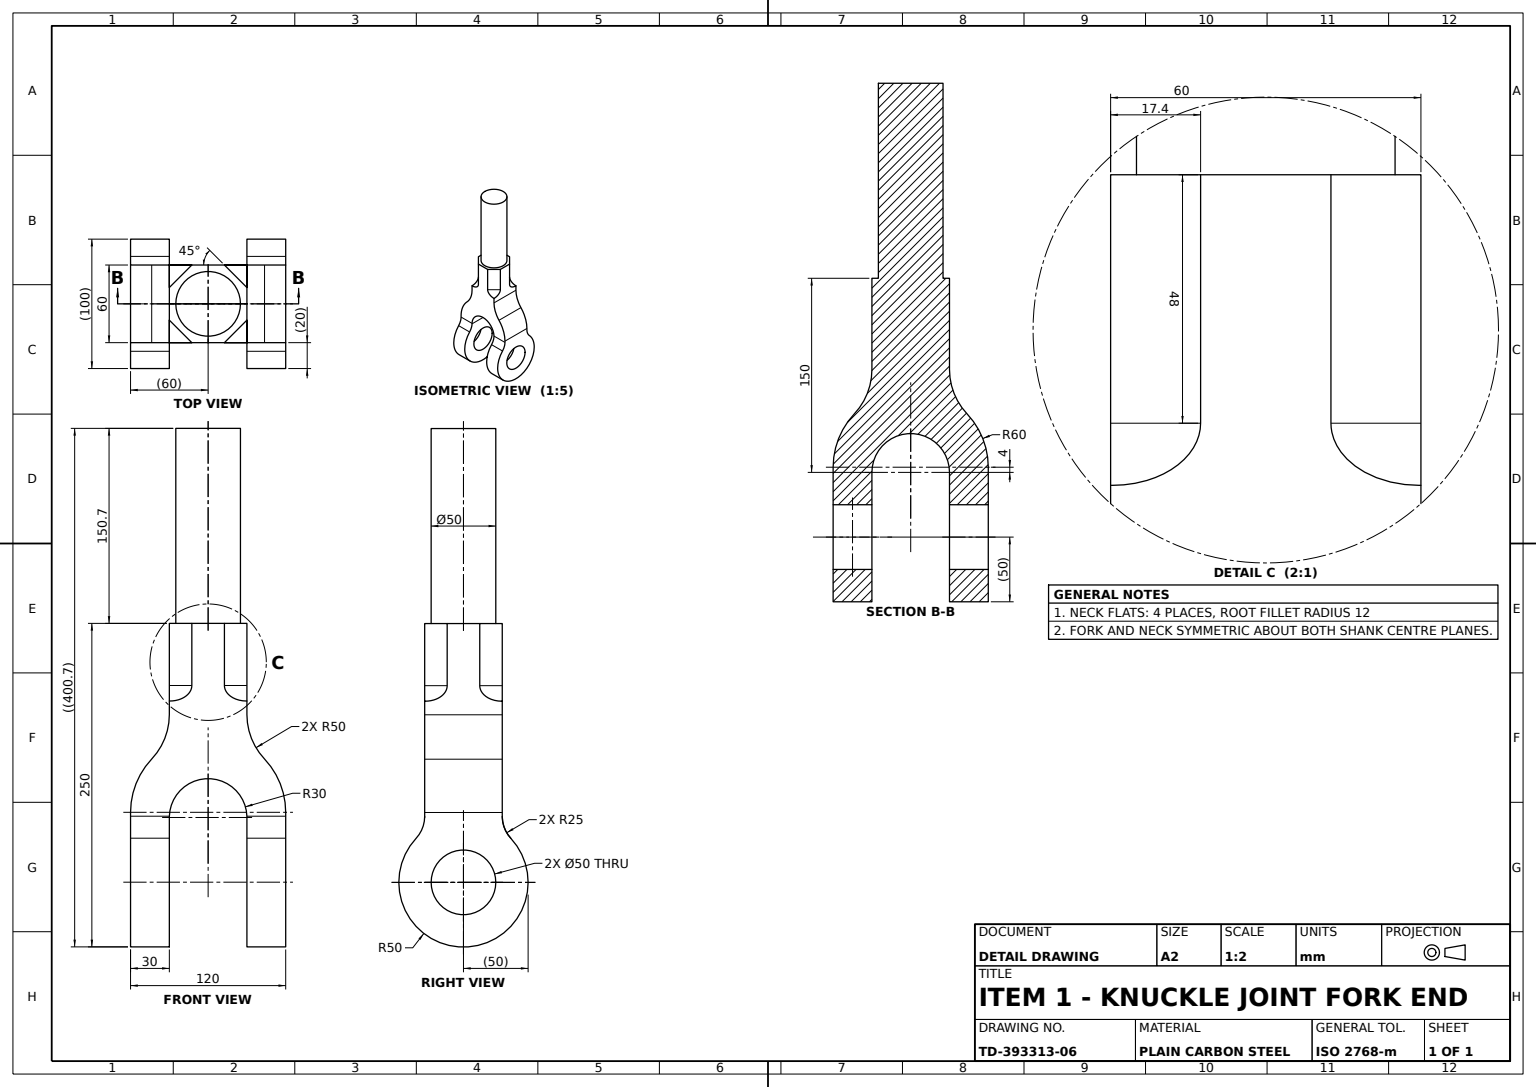
ISO-10303-21;
HEADER;
FILE_DESCRIPTION((''),'2;1');
FILE_NAME('','',(''),(''),'','','');
FILE_SCHEMA(('AUTOMOTIVE_DESIGN'));
ENDSEC;
DATA;
#1=APPLICATION_CONTEXT('');
#2=PRODUCT_CONTEXT('',#1,'mechanical');
#3=PRODUCT('','','',(#2));
#4=PRODUCT_DEFINITION_FORMATION('','',#3);
#5=PRODUCT_DEFINITION_CONTEXT('',#1,'design');
#6=PRODUCT_DEFINITION('','',#4,#5);
#7=PRODUCT_DEFINITION_SHAPE('','',#6);
#8=(LENGTH_UNIT()NAMED_UNIT(*)SI_UNIT(.MILLI.,.METRE.));
#9=(NAMED_UNIT(*)PLANE_ANGLE_UNIT()SI_UNIT($,.RADIAN.));
#10=(NAMED_UNIT(*)SI_UNIT($,.STERADIAN.)SOLID_ANGLE_UNIT());
#11=UNCERTAINTY_MEASURE_WITH_UNIT(LENGTH_MEASURE(1.E-05),#8,'distance_accuracy_value','');
#12=(GEOMETRIC_REPRESENTATION_CONTEXT(3)GLOBAL_UNCERTAINTY_ASSIGNED_CONTEXT((#11))GLOBAL_UNIT_ASSIGNED_CONTEXT((#8,#9,#10))REPRESENTATION_CONTEXT('',''));
#13=CARTESIAN_POINT('',(-90.,100.,19.980383));
#14=VERTEX_POINT('',#13);
#15=CARTESIAN_POINT('',(-90.,100.,80.019617));
#16=VERTEX_POINT('',#15);
#17=CARTESIAN_POINT('',(-90.,100.,0.));
#18=DIRECTION('',(0.,0.,1.));
#19=VECTOR('',#18,1000.);
#20=LINE('',#17,#19);
#21=EDGE_CURVE('',#14,#16,#20,.T.);
#22=ORIENTED_EDGE('',*,*,#21,.F.);
#23=CARTESIAN_POINT('',(-89.983654,100.990195,20.));
#24=VERTEX_POINT('',#23);
#25=CARTESIAN_POINT('',(-90.,100.164684,19.98691));
#26=CARTESIAN_POINT('',(-89.998644,100.329542,19.991814));
#27=CARTESIAN_POINT('',(-89.993202,100.659606,19.998359));
#28=CARTESIAN_POINT('',(-89.989107,100.825084,20.));
#29=B_SPLINE_CURVE_WITH_KNOTS('',3,(#13,#25,#26,#27,#28,#23),.UNSPECIFIED.,.F.,.F.,(4,2,4),(0.165848056,0.166335326,0.166822597),.UNSPECIFIED.);
#30=EDGE_CURVE('',#14,#24,#29,.T.);
#31=ORIENTED_EDGE('',*,*,#30,.T.);
#32=CARTESIAN_POINT('',(-30.016346,100.990195,20.));
#33=VERTEX_POINT('',#32);
#34=CARTESIAN_POINT('',(-60.,100.,20.));
#35=DIRECTION('',(0.,1.,0.));
#36=AXIS2_PLACEMENT_3D('',#34,#18,#35);
#37=CIRCLE('',#36,30.);
#38=EDGE_CURVE('',#33,#24,#37,.T.);
#39=ORIENTED_EDGE('',*,*,#38,.F.);
#40=CARTESIAN_POINT('',(-30.,100.,19.980383));
#41=VERTEX_POINT('',#40);
#42=CARTESIAN_POINT('',(-30.010903,100.82538,20.));
#43=CARTESIAN_POINT('',(-30.002731,100.495534,19.996741));
#44=CARTESIAN_POINT('',(-30.,100.165251,19.986933));
#45=B_SPLINE_CURVE_WITH_KNOTS('',3,(#32,#42,#43,#44,#40),.UNSPECIFIED.,.F.,.F.,(4,1,4),(0.085636646,0.086132211,0.086627775),.UNSPECIFIED.);
#46=EDGE_CURVE('',#33,#41,#45,.T.);
#47=ORIENTED_EDGE('',*,*,#46,.T.);
#48=CARTESIAN_POINT('',(-30.,100.,80.019617));
#49=VERTEX_POINT('',#48);
#50=CARTESIAN_POINT('',(-30.,100.,0.));
#51=LINE('',#50,#19);
#52=EDGE_CURVE('',#41,#49,#51,.T.);
#53=ORIENTED_EDGE('',*,*,#52,.T.);
#54=CARTESIAN_POINT('',(-30.016346,100.990195,80.));
#55=VERTEX_POINT('',#54);
#56=CARTESIAN_POINT('',(-30.005444,100.660091,80.));
#57=CARTESIAN_POINT('',(-30.,100.330025,80.006536));
#58=B_SPLINE_CURVE_WITH_KNOTS('',3,(#54,#56,#57,#48),.UNSPECIFIED.,.F.,.F.,(4,4),(0.,0.000990524),.UNSPECIFIED.);
#59=EDGE_CURVE('',#55,#49,#58,.T.);
#60=ORIENTED_EDGE('',*,*,#59,.F.);
#61=CARTESIAN_POINT('',(-89.983654,100.990195,80.));
#62=VERTEX_POINT('',#61);
#63=CARTESIAN_POINT('',(-60.,100.,80.));
#64=AXIS2_PLACEMENT_3D('',#63,#18,#35);
#65=CIRCLE('',#64,30.);
#66=EDGE_CURVE('',#55,#62,#65,.T.);
#67=ORIENTED_EDGE('',*,*,#66,.T.);
#68=CARTESIAN_POINT('',(-90.,100.330025,80.006536));
#69=CARTESIAN_POINT('',(-89.994556,100.660091,80.));
#70=B_SPLINE_CURVE_WITH_KNOTS('',3,(#15,#68,#69,#61),.UNSPECIFIED.,.F.,.F.,(4,4),(0.,0.000990524),.UNSPECIFIED.);
#71=EDGE_CURVE('',#16,#62,#70,.T.);
#72=ORIENTED_EDGE('',*,*,#71,.F.);
#73=EDGE_LOOP('',(#22,#31,#39,#47,#53,#60,#67,#72));
#74=FACE_OUTER_BOUND('',#73,.T.);
#75=CARTESIAN_POINT('',(-60.,100.,0.));
#76=DIRECTION('',(1.,0.,0.));
#77=AXIS2_PLACEMENT_3D('',#75,#18,#76);
#78=CYLINDRICAL_SURFACE('',#77,30.);
#79=ADVANCED_FACE('',(#74),#78,.F.);
#80=CARTESIAN_POINT('',(-120.,83.993463,86.666667));
#81=VERTEX_POINT('',#80);
#82=CARTESIAN_POINT('',(-120.,100.990195,80.));
#83=VERTEX_POINT('',#82);
#84=CARTESIAN_POINT('',(-120.,100.990195,105.));
#85=AXIS2_PLACEMENT_3D('',#84,#76,#18);
#86=CIRCLE('',#85,25.);
#87=EDGE_CURVE('',#81,#83,#86,.T.);
#88=ORIENTED_EDGE('',*,*,#87,.F.);
#89=CARTESIAN_POINT('',(-90.,83.993463,86.666667));
#90=VERTEX_POINT('',#89);
#91=CARTESIAN_POINT('',(0.,83.993463,86.666667));
#92=DIRECTION('',(-1.,0.,0.));
#93=VECTOR('',#92,1000.);
#94=LINE('',#91,#93);
#95=EDGE_CURVE('',#90,#81,#94,.T.);
#96=ORIENTED_EDGE('',*,*,#95,.F.);
#97=CARTESIAN_POINT('',(-90.,100.990195,105.));
#98=DIRECTION('',(0.,-1.,0.));
#99=AXIS2_PLACEMENT_3D('',#97,#76,#98);
#100=CIRCLE('',#99,25.);
#101=EDGE_CURVE('',#90,#16,#100,.T.);
#102=ORIENTED_EDGE('',*,*,#101,.T.);
#103=ORIENTED_EDGE('',*,*,#71,.T.);
#104=CARTESIAN_POINT('',(0.,100.990195,80.));
#105=LINE('',#104,#93);
#106=EDGE_CURVE('',#62,#83,#105,.T.);
#107=ORIENTED_EDGE('',*,*,#106,.T.);
#108=EDGE_LOOP('',(#88,#96,#102,#103,#107));
#109=FACE_OUTER_BOUND('',#108,.T.);
#110=CARTESIAN_POINT('',(0.,100.990195,105.));
#111=AXIS2_PLACEMENT_3D('',#110,#92,#18);
#112=CYLINDRICAL_SURFACE('',#111,25.);
#113=ADVANCED_FACE('',(#109),#112,.F.);
#114=CARTESIAN_POINT('',(-120.,50.,0.));
#115=VERTEX_POINT('',#114);
#116=CARTESIAN_POINT('',(-120.,50.,100.));
#117=VERTEX_POINT('',#116);
#118=CARTESIAN_POINT('',(-120.,50.,50.));
#119=AXIS2_PLACEMENT_3D('',#118,#92,#18);
#120=CIRCLE('',#119,50.);
#121=EDGE_CURVE('',#115,#117,#120,.T.);
#122=ORIENTED_EDGE('',*,*,#121,.T.);
#123=EDGE_CURVE('',#117,#81,#120,.T.);
#124=ORIENTED_EDGE('',*,*,#123,.T.);
#125=ORIENTED_EDGE('',*,*,#87,.T.);
#126=CARTESIAN_POINT('',(-120.,104.,80.));
#127=VERTEX_POINT('',#126);
#128=CARTESIAN_POINT('',(-120.,0.,80.));
#129=VECTOR('',#98,1000.);
#130=LINE('',#128,#129);
#131=EDGE_CURVE('',#127,#83,#130,.T.);
#132=ORIENTED_EDGE('',*,*,#131,.F.);
#133=CARTESIAN_POINT('',(-120.,104.,20.));
#134=VERTEX_POINT('',#133);
#135=CARTESIAN_POINT('',(-120.,104.,0.));
#136=LINE('',#135,#19);
#137=EDGE_CURVE('',#134,#127,#136,.T.);
#138=ORIENTED_EDGE('',*,*,#137,.F.);
#139=CARTESIAN_POINT('',(-120.,100.990195,20.));
#140=VERTEX_POINT('',#139);
#141=CARTESIAN_POINT('',(-120.,0.,20.));
#142=LINE('',#141,#129);
#143=EDGE_CURVE('',#134,#140,#142,.T.);
#144=ORIENTED_EDGE('',*,*,#143,.T.);
#145=CARTESIAN_POINT('',(-120.,83.993463,13.333333));
#146=VERTEX_POINT('',#145);
#147=CARTESIAN_POINT('',(-120.,100.990195,-5.));
#148=AXIS2_PLACEMENT_3D('',#147,#92,#18);
#149=CIRCLE('',#148,25.);
#150=EDGE_CURVE('',#146,#140,#149,.T.);
#151=ORIENTED_EDGE('',*,*,#150,.F.);
#152=EDGE_CURVE('',#146,#115,#120,.T.);
#153=ORIENTED_EDGE('',*,*,#152,.T.);
#154=EDGE_LOOP('',(#122,#124,#125,#132,#138,#144,#151,#153));
#155=FACE_OUTER_BOUND('',#154,.T.);
#156=CARTESIAN_POINT('',(-120.,50.,25.));
#157=VERTEX_POINT('',#156);
#158=CARTESIAN_POINT('',(-120.,50.,75.));
#159=VERTEX_POINT('',#158);
#160=CIRCLE('',#119,25.);
#161=EDGE_CURVE('',#157,#159,#160,.T.);
#162=ORIENTED_EDGE('',*,*,#161,.F.);
#163=EDGE_CURVE('',#159,#157,#160,.T.);
#164=ORIENTED_EDGE('',*,*,#163,.F.);
#165=EDGE_LOOP('',(#162,#164));
#166=FACE_BOUND('',#165,.T.);
#167=CARTESIAN_POINT('',(-120.,0.,100.));
#168=DIRECTION('',(0.,0.,-1.));
#169=AXIS2_PLACEMENT_3D('',#167,#76,#168);
#170=PLANE('',#169);
#171=ADVANCED_FACE('',(#155,#166),#170,.F.);
#172=CARTESIAN_POINT('',(-30.,250.,37.4));
#173=VERTEX_POINT('',#172);
#174=CARTESIAN_POINT('',(-47.4,250.,20.));
#175=VERTEX_POINT('',#174);
#176=CARTESIAN_POINT('',(-33.7,250.,33.7));
#177=DIRECTION('',(-0.707106781,0.,-0.707106781));
#178=VECTOR('',#177,1000.);
#179=LINE('',#176,#178);
#180=EDGE_CURVE('',#173,#175,#179,.T.);
#181=ORIENTED_EDGE('',*,*,#180,.F.);
#182=CARTESIAN_POINT('',(-30.,202.,37.4));
#183=VERTEX_POINT('',#182);
#184=CARTESIAN_POINT('',(-30.,190.,37.4));
#185=VECTOR('',#35,1000.);
#186=LINE('',#184,#185);
#187=EDGE_CURVE('',#183,#173,#186,.T.);
#188=ORIENTED_EDGE('',*,*,#187,.F.);
#189=CARTESIAN_POINT('',(-47.4,202.,20.));
#190=VERTEX_POINT('',#189);
#191=LINE('',#189,#178);
#192=EDGE_CURVE('',#183,#190,#191,.T.);
#193=ORIENTED_EDGE('',*,*,#192,.T.);
#194=CARTESIAN_POINT('',(-47.4,190.,20.));
#195=LINE('',#194,#185);
#196=EDGE_CURVE('',#190,#175,#195,.T.);
#197=ORIENTED_EDGE('',*,*,#196,.T.);
#198=EDGE_LOOP('',(#181,#188,#193,#197));
#199=FACE_OUTER_BOUND('',#198,.T.);
#200=CARTESIAN_POINT('',(-33.7,190.,33.7));
#201=DIRECTION('',(0.707106781,0.,-0.707106781));
#202=AXIS2_PLACEMENT_3D('',#200,#201,#177);
#203=PLANE('',#202);
#204=ADVANCED_FACE('',(#199),#203,.T.);
#205=CARTESIAN_POINT('',(-90.,50.,75.));
#206=VERTEX_POINT('',#205);
#207=CARTESIAN_POINT('',(0.,50.,75.));
#208=LINE('',#207,#93);
#209=EDGE_CURVE('',#206,#159,#208,.T.);
#210=ORIENTED_EDGE('',*,*,#209,.F.);
#211=CARTESIAN_POINT('',(-90.,50.,25.));
#212=VERTEX_POINT('',#211);
#213=CARTESIAN_POINT('',(-90.,50.,50.));
#214=AXIS2_PLACEMENT_3D('',#213,#92,#98);
#215=CIRCLE('',#214,25.);
#216=EDGE_CURVE('',#212,#206,#215,.T.);
#217=ORIENTED_EDGE('',*,*,#216,.F.);
#218=CARTESIAN_POINT('',(0.,50.,25.));
#219=LINE('',#218,#93);
#220=EDGE_CURVE('',#212,#157,#219,.T.);
#221=ORIENTED_EDGE('',*,*,#220,.T.);
#222=ORIENTED_EDGE('',*,*,#161,.T.);
#223=EDGE_LOOP('',(#210,#217,#221,#222));
#224=FACE_OUTER_BOUND('',#223,.T.);
#225=CARTESIAN_POINT('',(0.,50.,50.));
#226=AXIS2_PLACEMENT_3D('',#225,#92,#18);
#227=CYLINDRICAL_SURFACE('',#226,25.);
#228=ADVANCED_FACE('',(#224),#227,.F.);
#229=EDGE_CURVE('',#206,#212,#215,.T.);
#230=ORIENTED_EDGE('',*,*,#229,.F.);
#231=ORIENTED_EDGE('',*,*,#209,.T.);
#232=ORIENTED_EDGE('',*,*,#163,.T.);
#233=ORIENTED_EDGE('',*,*,#220,.F.);
#234=EDGE_LOOP('',(#230,#231,#232,#233));
#235=FACE_OUTER_BOUND('',#234,.T.);
#236=ADVANCED_FACE('',(#235),#227,.F.);
#237=CARTESIAN_POINT('',(-90.,83.993463,13.333333));
#238=VERTEX_POINT('',#237);
#239=CARTESIAN_POINT('',(-90.,100.990195,-5.));
#240=AXIS2_PLACEMENT_3D('',#239,#92,#98);
#241=CIRCLE('',#240,25.);
#242=EDGE_CURVE('',#238,#14,#241,.T.);
#243=ORIENTED_EDGE('',*,*,#242,.F.);
#244=CARTESIAN_POINT('',(0.,83.993463,13.333333));
#245=LINE('',#244,#93);
#246=EDGE_CURVE('',#238,#146,#245,.T.);
#247=ORIENTED_EDGE('',*,*,#246,.T.);
#248=ORIENTED_EDGE('',*,*,#150,.T.);
#249=CARTESIAN_POINT('',(0.,100.990195,20.));
#250=LINE('',#249,#93);
#251=EDGE_CURVE('',#24,#140,#250,.T.);
#252=ORIENTED_EDGE('',*,*,#251,.F.);
#253=ORIENTED_EDGE('',*,*,#30,.F.);
#254=EDGE_LOOP('',(#243,#247,#248,#252,#253));
#255=FACE_OUTER_BOUND('',#254,.T.);
#256=CARTESIAN_POINT('',(0.,100.990195,-5.));
#257=AXIS2_PLACEMENT_3D('',#256,#92,#18);
#258=CYLINDRICAL_SURFACE('',#257,25.);
#259=ADVANCED_FACE('',(#255),#258,.F.);
#260=CARTESIAN_POINT('',(-47.4,202.,80.));
#261=VERTEX_POINT('',#260);
#262=CARTESIAN_POINT('',(-30.,202.,62.6));
#263=VERTEX_POINT('',#262);
#264=VECTOR('',#201,1000.);
#265=LINE('',#262,#264);
#266=EDGE_CURVE('',#261,#263,#265,.T.);
#267=ORIENTED_EDGE('',*,*,#266,.F.);
#268=CARTESIAN_POINT('',(-30.429437,190.,80.));
#269=VERTEX_POINT('',#268);
#270=CARTESIAN_POINT('',(-40.370563,190.,80.));
#271=CARTESIAN_POINT('',(-47.4,194.970563,80.));
#272=(BOUNDED_CURVE()B_SPLINE_CURVE(3,(#268,#270,#271,#260),.UNSPECIFIED.,.F.,.F.)B_SPLINE_CURVE_WITH_KNOTS((4,4),(4.71238898,6.283185307),.UNSPECIFIED.)CURVE()GEOMETRIC_REPRESENTATION_ITEM()RATIONAL_B_SPLINE_CURVE((1.,0.804737854,0.804737854,1.))REPRESENTATION_ITEM(''));
#273=EDGE_CURVE('',#269,#261,#272,.T.);
#274=ORIENTED_EDGE('',*,*,#273,.F.);
#275=CARTESIAN_POINT('',(-30.,190.,79.570563));
#276=VERTEX_POINT('',#275);
#277=CARTESIAN_POINT('',(-38.914719,190.,88.485281));
#278=DIRECTION('',(-0.707106781,0.,0.707106781));
#279=VECTOR('',#278,1000.);
#280=LINE('',#277,#279);
#281=EDGE_CURVE('',#276,#269,#280,.T.);
#282=ORIENTED_EDGE('',*,*,#281,.F.);
#283=CARTESIAN_POINT('',(-30.,194.970563,62.6));
#284=CARTESIAN_POINT('',(-30.,190.,69.629437));
#285=(BOUNDED_CURVE()B_SPLINE_CURVE(3,(#262,#283,#284,#275),.UNSPECIFIED.,.F.,.F.)B_SPLINE_CURVE_WITH_KNOTS((4,4),(3.141592654,4.71238898),.UNSPECIFIED.)CURVE()GEOMETRIC_REPRESENTATION_ITEM()RATIONAL_B_SPLINE_CURVE((1.,0.804737854,0.804737854,1.))REPRESENTATION_ITEM(''));
#286=EDGE_CURVE('',#263,#276,#285,.T.);
#287=ORIENTED_EDGE('',*,*,#286,.F.);
#288=EDGE_LOOP('',(#267,#274,#282,#287));
#289=FACE_OUTER_BOUND('',#288,.T.);
#290=CARTESIAN_POINT('',(24.785281,202.,24.785281));
#291=DIRECTION('',(0.707106781,0.,0.707106781));
#292=AXIS2_PLACEMENT_3D('',#290,#278,#291);
#293=CYLINDRICAL_SURFACE('',#292,12.);
#294=ADVANCED_FACE('',(#289),#293,.F.);
#295=CARTESIAN_POINT('',(-35.,400.7,50.));
#296=VERTEX_POINT('',#295);
#297=CARTESIAN_POINT('',(-85.,400.7,50.));
#298=VERTEX_POINT('',#297);
#299=CARTESIAN_POINT('',(-60.,400.7,50.));
#300=AXIS2_PLACEMENT_3D('',#299,#35,#92);
#301=CIRCLE('',#300,25.);
#302=EDGE_CURVE('',#296,#298,#301,.T.);
#303=ORIENTED_EDGE('',*,*,#302,.F.);
#304=CARTESIAN_POINT('',(-35.,250.,50.));
#305=VERTEX_POINT('',#304);
#306=LINE('',#295,#129);
#307=EDGE_CURVE('',#296,#305,#306,.T.);
#308=ORIENTED_EDGE('',*,*,#307,.T.);
#309=CARTESIAN_POINT('',(-85.,250.,50.));
#310=VERTEX_POINT('',#309);
#311=CARTESIAN_POINT('',(-60.,250.,50.));
#312=AXIS2_PLACEMENT_3D('',#311,#35,#92);
#313=CIRCLE('',#312,25.);
#314=EDGE_CURVE('',#305,#310,#313,.T.);
#315=ORIENTED_EDGE('',*,*,#314,.T.);
#316=LINE('',#297,#129);
#317=EDGE_CURVE('',#298,#310,#316,.T.);
#318=ORIENTED_EDGE('',*,*,#317,.F.);
#319=EDGE_LOOP('',(#303,#308,#315,#318));
#320=FACE_OUTER_BOUND('',#319,.T.);
#321=AXIS2_PLACEMENT_3D('',#299,#98,#76);
#322=CYLINDRICAL_SURFACE('',#321,25.);
#323=ADVANCED_FACE('',(#320),#322,.T.);
#324=CARTESIAN_POINT('',(-90.,190.,79.570563));
#325=VERTEX_POINT('',#324);
#326=CARTESIAN_POINT('',(-90.,190.,80.));
#327=VERTEX_POINT('',#326);
#328=CARTESIAN_POINT('',(-90.,190.,0.));
#329=LINE('',#328,#19);
#330=EDGE_CURVE('',#325,#327,#329,.T.);
#331=ORIENTED_EDGE('',*,*,#330,.T.);
#332=CARTESIAN_POINT('',(-89.570563,190.,80.));
#333=VERTEX_POINT('',#332);
#334=CARTESIAN_POINT('',(0.,190.,80.));
#335=VECTOR('',#76,1000.);
#336=LINE('',#334,#335);
#337=EDGE_CURVE('',#327,#333,#336,.T.);
#338=ORIENTED_EDGE('',*,*,#337,.T.);
#339=CARTESIAN_POINT('',(-98.485281,190.,71.085281));
#340=LINE('',#339,#178);
#341=EDGE_CURVE('',#333,#325,#340,.T.);
#342=ORIENTED_EDGE('',*,*,#341,.T.);
#343=EDGE_LOOP('',(#331,#338,#342));
#344=FACE_OUTER_BOUND('',#343,.T.);
#345=CARTESIAN_POINT('',(0.,190.,0.));
#346=AXIS2_PLACEMENT_3D('',#345,#35,#92);
#347=PLANE('',#346);
#348=ADVANCED_FACE('',(#344),#347,.T.);
#349=CARTESIAN_POINT('',(-90.,190.,20.429437));
#350=VERTEX_POINT('',#349);
#351=CARTESIAN_POINT('',(-89.570563,190.,20.));
#352=VERTEX_POINT('',#351);
#353=CARTESIAN_POINT('',(-81.085281,190.,11.514719));
#354=LINE('',#353,#264);
#355=EDGE_CURVE('',#350,#352,#354,.T.);
#356=ORIENTED_EDGE('',*,*,#355,.T.);
#357=CARTESIAN_POINT('',(-90.,190.,20.));
#358=VERTEX_POINT('',#357);
#359=CARTESIAN_POINT('',(0.,190.,20.));
#360=LINE('',#359,#93);
#361=EDGE_CURVE('',#352,#358,#360,.T.);
#362=ORIENTED_EDGE('',*,*,#361,.T.);
#363=EDGE_CURVE('',#358,#350,#329,.T.);
#364=ORIENTED_EDGE('',*,*,#363,.T.);
#365=EDGE_LOOP('',(#356,#362,#364));
#366=FACE_OUTER_BOUND('',#365,.T.);
#367=ADVANCED_FACE('',(#366),#347,.T.);
#368=ORIENTED_EDGE('',*,*,#281,.T.);
#369=CARTESIAN_POINT('',(-30.,190.,80.));
#370=VERTEX_POINT('',#369);
#371=EDGE_CURVE('',#269,#370,#336,.T.);
#372=ORIENTED_EDGE('',*,*,#371,.T.);
#373=CARTESIAN_POINT('',(-30.,190.,0.));
#374=VECTOR('',#168,1000.);
#375=LINE('',#373,#374);
#376=EDGE_CURVE('',#370,#276,#375,.T.);
#377=ORIENTED_EDGE('',*,*,#376,.T.);
#378=EDGE_LOOP('',(#368,#372,#377));
#379=FACE_OUTER_BOUND('',#378,.T.);
#380=ADVANCED_FACE('',(#379),#347,.T.);
#381=ORIENTED_EDGE('',*,*,#46,.F.);
#382=VERTEX_POINT('',#249);
#383=EDGE_CURVE('',#382,#33,#250,.T.);
#384=ORIENTED_EDGE('',*,*,#383,.F.);
#385=VERTEX_POINT('',#244);
#386=CIRCLE('',#257,25.);
#387=EDGE_CURVE('',#385,#382,#386,.T.);
#388=ORIENTED_EDGE('',*,*,#387,.F.);
#389=CARTESIAN_POINT('',(-30.,83.993463,13.333333));
#390=VERTEX_POINT('',#389);
#391=EDGE_CURVE('',#385,#390,#245,.T.);
#392=ORIENTED_EDGE('',*,*,#391,.T.);
#393=CARTESIAN_POINT('',(-30.,100.990195,-5.));
#394=AXIS2_PLACEMENT_3D('',#393,#92,#98);
#395=CIRCLE('',#394,25.);
#396=EDGE_CURVE('',#390,#41,#395,.T.);
#397=ORIENTED_EDGE('',*,*,#396,.T.);
#398=EDGE_LOOP('',(#381,#384,#388,#392,#397));
#399=FACE_OUTER_BOUND('',#398,.T.);
#400=ADVANCED_FACE('',(#399),#258,.F.);
#401=CARTESIAN_POINT('',(-30.,50.,25.));
#402=VERTEX_POINT('',#401);
#403=CARTESIAN_POINT('',(-30.,50.,75.));
#404=VERTEX_POINT('',#403);
#405=CARTESIAN_POINT('',(-30.,50.,50.));
#406=AXIS2_PLACEMENT_3D('',#405,#92,#98);
#407=CIRCLE('',#406,25.);
#408=EDGE_CURVE('',#402,#404,#407,.T.);
#409=ORIENTED_EDGE('',*,*,#408,.F.);
#410=EDGE_CURVE('',#404,#402,#407,.T.);
#411=ORIENTED_EDGE('',*,*,#410,.F.);
#412=EDGE_LOOP('',(#409,#411));
#413=FACE_BOUND('',#412,.T.);
#414=CARTESIAN_POINT('',(-30.,50.,0.));
#415=VERTEX_POINT('',#414);
#416=CIRCLE('',#406,50.);
#417=EDGE_CURVE('',#390,#415,#416,.T.);
#418=ORIENTED_EDGE('',*,*,#417,.T.);
#419=CARTESIAN_POINT('',(-30.,50.,100.));
#420=VERTEX_POINT('',#419);
#421=EDGE_CURVE('',#415,#420,#416,.T.);
#422=ORIENTED_EDGE('',*,*,#421,.T.);
#423=CARTESIAN_POINT('',(-30.,83.993463,86.666667));
#424=VERTEX_POINT('',#423);
#425=EDGE_CURVE('',#420,#424,#416,.T.);
#426=ORIENTED_EDGE('',*,*,#425,.T.);
#427=CARTESIAN_POINT('',(-30.,100.990195,105.));
#428=AXIS2_PLACEMENT_3D('',#427,#76,#98);
#429=CIRCLE('',#428,25.);
#430=EDGE_CURVE('',#424,#49,#429,.T.);
#431=ORIENTED_EDGE('',*,*,#430,.T.);
#432=ORIENTED_EDGE('',*,*,#52,.F.);
#433=ORIENTED_EDGE('',*,*,#396,.F.);
#434=EDGE_LOOP('',(#418,#422,#426,#431,#432,#433));
#435=FACE_OUTER_BOUND('',#434,.T.);
#436=CARTESIAN_POINT('',(-30.,0.,0.));
#437=AXIS2_PLACEMENT_3D('',#436,#92,#98);
#438=PLANE('',#437);
#439=ADVANCED_FACE('',(#413,#435),#438,.T.);
#440=CARTESIAN_POINT('',(-90.,50.,0.));
#441=VERTEX_POINT('',#440);
#442=CARTESIAN_POINT('',(0.,50.,0.));
#443=LINE('',#442,#93);
#444=EDGE_CURVE('',#441,#115,#443,.T.);
#445=ORIENTED_EDGE('',*,*,#444,.F.);
#446=CARTESIAN_POINT('',(-90.,50.,100.));
#447=VERTEX_POINT('',#446);
#448=CIRCLE('',#214,50.);
#449=EDGE_CURVE('',#441,#447,#448,.T.);
#450=ORIENTED_EDGE('',*,*,#449,.T.);
#451=CARTESIAN_POINT('',(0.,50.,100.));
#452=LINE('',#451,#93);
#453=EDGE_CURVE('',#447,#117,#452,.T.);
#454=ORIENTED_EDGE('',*,*,#453,.T.);
#455=ORIENTED_EDGE('',*,*,#121,.F.);
#456=EDGE_LOOP('',(#445,#450,#454,#455));
#457=FACE_OUTER_BOUND('',#456,.T.);
#458=CYLINDRICAL_SURFACE('',#226,50.);
#459=ADVANCED_FACE('',(#457),#458,.T.);
#460=ORIENTED_EDGE('',*,*,#408,.T.);
#461=VERTEX_POINT('',#207);
#462=EDGE_CURVE('',#461,#404,#208,.T.);
#463=ORIENTED_EDGE('',*,*,#462,.F.);
#464=VERTEX_POINT('',#218);
#465=CIRCLE('',#226,25.);
#466=EDGE_CURVE('',#464,#461,#465,.T.);
#467=ORIENTED_EDGE('',*,*,#466,.F.);
#468=EDGE_CURVE('',#464,#402,#219,.T.);
#469=ORIENTED_EDGE('',*,*,#468,.T.);
#470=EDGE_LOOP('',(#460,#463,#467,#469));
#471=FACE_OUTER_BOUND('',#470,.T.);
#472=ADVANCED_FACE('',(#471),#227,.F.);
#473=VERTEX_POINT('',#442);
#474=EDGE_CURVE('',#473,#415,#443,.T.);
#475=ORIENTED_EDGE('',*,*,#474,.F.);
#476=VERTEX_POINT('',#451);
#477=CIRCLE('',#226,50.);
#478=EDGE_CURVE('',#473,#476,#477,.T.);
#479=ORIENTED_EDGE('',*,*,#478,.T.);
#480=EDGE_CURVE('',#476,#420,#452,.T.);
#481=ORIENTED_EDGE('',*,*,#480,.T.);
#482=ORIENTED_EDGE('',*,*,#421,.F.);
#483=EDGE_LOOP('',(#475,#479,#481,#482));
#484=FACE_OUTER_BOUND('',#483,.T.);
#485=ADVANCED_FACE('',(#484),#458,.T.);
#486=VERTEX_POINT('',#91);
#487=VERTEX_POINT('',#104);
#488=AXIS2_PLACEMENT_3D('',#110,#76,#18);
#489=CIRCLE('',#488,25.);
#490=EDGE_CURVE('',#486,#487,#489,.T.);
#491=ORIENTED_EDGE('',*,*,#490,.T.);
#492=EDGE_CURVE('',#487,#55,#105,.T.);
#493=ORIENTED_EDGE('',*,*,#492,.T.);
#494=ORIENTED_EDGE('',*,*,#59,.T.);
#495=ORIENTED_EDGE('',*,*,#430,.F.);
#496=EDGE_CURVE('',#486,#424,#94,.T.);
#497=ORIENTED_EDGE('',*,*,#496,.F.);
#498=EDGE_LOOP('',(#491,#493,#494,#495,#497));
#499=FACE_OUTER_BOUND('',#498,.T.);
#500=ADVANCED_FACE('',(#499),#112,.F.);
#501=CARTESIAN_POINT('',(-30.,179.498344,80.));
#502=VERTEX_POINT('',#501);
#503=CARTESIAN_POINT('',(-16.363636,145.180915,80.));
#504=VERTEX_POINT('',#503);
#505=CARTESIAN_POINT('',(20.,179.498344,80.));
#506=AXIS2_PLACEMENT_3D('',#505,#18,#35);
#507=CIRCLE('',#506,50.);
#508=EDGE_CURVE('',#502,#504,#507,.T.);
#509=ORIENTED_EDGE('',*,*,#508,.F.);
#510=CARTESIAN_POINT('',(-30.,0.,80.));
#511=LINE('',#510,#129);
#512=EDGE_CURVE('',#370,#502,#511,.T.);
#513=ORIENTED_EDGE('',*,*,#512,.F.);
#514=ORIENTED_EDGE('',*,*,#371,.F.);
#515=ORIENTED_EDGE('',*,*,#273,.T.);
#516=CARTESIAN_POINT('',(-47.4,250.,80.));
#517=VERTEX_POINT('',#516);
#518=CARTESIAN_POINT('',(-47.4,190.,80.));
#519=LINE('',#518,#185);
#520=EDGE_CURVE('',#261,#517,#519,.T.);
#521=ORIENTED_EDGE('',*,*,#520,.T.);
#522=CARTESIAN_POINT('',(-72.6,250.,80.));
#523=VERTEX_POINT('',#522);
#524=CARTESIAN_POINT('',(0.,250.,80.));
#525=LINE('',#524,#93);
#526=EDGE_CURVE('',#517,#523,#525,.T.);
#527=ORIENTED_EDGE('',*,*,#526,.T.);
#528=CARTESIAN_POINT('',(-72.6,202.,80.));
#529=VERTEX_POINT('',#528);
#530=CARTESIAN_POINT('',(-72.6,190.,80.));
#531=LINE('',#530,#185);
#532=EDGE_CURVE('',#529,#523,#531,.T.);
#533=ORIENTED_EDGE('',*,*,#532,.F.);
#534=CARTESIAN_POINT('',(-72.6,194.970563,80.));
#535=CARTESIAN_POINT('',(-79.629437,190.,80.));
#536=(BOUNDED_CURVE()B_SPLINE_CURVE(3,(#528,#534,#535,#332),.UNSPECIFIED.,.F.,.T.)B_SPLINE_CURVE_WITH_KNOTS((4,4),(3.141592654,4.71238898),.UNSPECIFIED.)CURVE()GEOMETRIC_REPRESENTATION_ITEM()RATIONAL_B_SPLINE_CURVE((1.,0.804737854,0.804737854,1.))REPRESENTATION_ITEM(''));
#537=EDGE_CURVE('',#529,#333,#536,.T.);
#538=ORIENTED_EDGE('',*,*,#537,.T.);
#539=ORIENTED_EDGE('',*,*,#337,.F.);
#540=CARTESIAN_POINT('',(-90.,179.498344,80.));
#541=VERTEX_POINT('',#540);
#542=CARTESIAN_POINT('',(-90.,0.,80.));
#543=LINE('',#542,#129);
#544=EDGE_CURVE('',#327,#541,#543,.T.);
#545=ORIENTED_EDGE('',*,*,#544,.T.);
#546=CARTESIAN_POINT('',(-103.636364,145.180915,80.));
#547=VERTEX_POINT('',#546);
#548=CARTESIAN_POINT('',(-140.,179.498344,80.));
#549=AXIS2_PLACEMENT_3D('',#548,#168,#35);
#550=CIRCLE('',#549,50.);
#551=EDGE_CURVE('',#541,#547,#550,.T.);
#552=ORIENTED_EDGE('',*,*,#551,.T.);
#553=CARTESIAN_POINT('',(-60.,104.,80.));
#554=AXIS2_PLACEMENT_3D('',#553,#18,#35);
#555=CIRCLE('',#554,60.);
#556=EDGE_CURVE('',#547,#127,#555,.T.);
#557=ORIENTED_EDGE('',*,*,#556,.T.);
#558=ORIENTED_EDGE('',*,*,#131,.T.);
#559=ORIENTED_EDGE('',*,*,#106,.F.);
#560=ORIENTED_EDGE('',*,*,#66,.F.);
#561=ORIENTED_EDGE('',*,*,#492,.F.);
#562=CARTESIAN_POINT('',(0.,104.,80.));
#563=VERTEX_POINT('',#562);
#564=CARTESIAN_POINT('',(0.,0.,80.));
#565=LINE('',#564,#129);
#566=EDGE_CURVE('',#563,#487,#565,.T.);
#567=ORIENTED_EDGE('',*,*,#566,.F.);
#568=EDGE_CURVE('',#563,#504,#555,.T.);
#569=ORIENTED_EDGE('',*,*,#568,.T.);
#570=EDGE_LOOP('',(#509,#513,#514,#515,#521,#527,#533,#538,#539,#545,#552,#557,#558,#559,#560,#561,#567,#569));
#571=FACE_OUTER_BOUND('',#570,.T.);
#572=AXIS2_PLACEMENT_3D('',#564,#168,#35);
#573=PLANE('',#572);
#574=ADVANCED_FACE('',(#571),#573,.F.);
#575=CARTESIAN_POINT('',(-16.363636,145.180915,20.));
#576=VERTEX_POINT('',#575);
#577=CARTESIAN_POINT('',(-16.363636,145.180915,0.));
#578=LINE('',#577,#19);
#579=EDGE_CURVE('',#576,#504,#578,.T.);
#580=ORIENTED_EDGE('',*,*,#579,.T.);
#581=ORIENTED_EDGE('',*,*,#568,.F.);
#582=CARTESIAN_POINT('',(0.,104.,20.));
#583=VERTEX_POINT('',#582);
#584=CARTESIAN_POINT('',(0.,104.,0.));
#585=LINE('',#584,#19);
#586=EDGE_CURVE('',#583,#563,#585,.T.);
#587=ORIENTED_EDGE('',*,*,#586,.F.);
#588=CARTESIAN_POINT('',(-60.,104.,20.));
#589=AXIS2_PLACEMENT_3D('',#588,#18,#35);
#590=CIRCLE('',#589,60.);
#591=EDGE_CURVE('',#583,#576,#590,.T.);
#592=ORIENTED_EDGE('',*,*,#591,.T.);
#593=EDGE_LOOP('',(#580,#581,#587,#592));
#594=FACE_OUTER_BOUND('',#593,.T.);
#595=CARTESIAN_POINT('',(-60.,104.,0.));
#596=AXIS2_PLACEMENT_3D('',#595,#18,#76);
#597=CYLINDRICAL_SURFACE('',#596,60.);
#598=ADVANCED_FACE('',(#594),#597,.T.);
#599=CARTESIAN_POINT('',(-72.6,202.,20.));
#600=VERTEX_POINT('',#599);
#601=CARTESIAN_POINT('',(-79.629437,190.,20.));
#602=CARTESIAN_POINT('',(-72.6,194.970563,20.));
#603=(BOUNDED_CURVE()B_SPLINE_CURVE(3,(#351,#601,#602,#599),.UNSPECIFIED.,.F.,.F.)B_SPLINE_CURVE_WITH_KNOTS((4,4),(4.71238898,6.283185307),.UNSPECIFIED.)CURVE()GEOMETRIC_REPRESENTATION_ITEM()RATIONAL_B_SPLINE_CURVE((1.,0.804737854,0.804737854,1.))REPRESENTATION_ITEM(''));
#604=EDGE_CURVE('',#352,#600,#603,.T.);
#605=ORIENTED_EDGE('',*,*,#604,.F.);
#606=ORIENTED_EDGE('',*,*,#355,.F.);
#607=CARTESIAN_POINT('',(-90.,202.,37.4));
#608=VERTEX_POINT('',#607);
#609=CARTESIAN_POINT('',(-90.,194.970563,37.4));
#610=CARTESIAN_POINT('',(-90.,190.,30.370563));
#611=(BOUNDED_CURVE()B_SPLINE_CURVE(3,(#607,#609,#610,#349),.UNSPECIFIED.,.F.,.T.)B_SPLINE_CURVE_WITH_KNOTS((4,4),(3.141592654,4.71238898),.UNSPECIFIED.)CURVE()GEOMETRIC_REPRESENTATION_ITEM()RATIONAL_B_SPLINE_CURVE((1.,0.804737854,0.804737854,1.))REPRESENTATION_ITEM(''));
#612=EDGE_CURVE('',#608,#350,#611,.T.);
#613=ORIENTED_EDGE('',*,*,#612,.F.);
#614=LINE('',#607,#279);
#615=EDGE_CURVE('',#600,#608,#614,.T.);
#616=ORIENTED_EDGE('',*,*,#615,.F.);
#617=EDGE_LOOP('',(#605,#606,#613,#616));
#618=FACE_OUTER_BOUND('',#617,.T.);
#619=CARTESIAN_POINT('',(-34.785281,202.,-34.785281));
#620=AXIS2_PLACEMENT_3D('',#619,#201,#177);
#621=CYLINDRICAL_SURFACE('',#620,12.);
#622=ADVANCED_FACE('',(#618),#621,.F.);
#623=ORIENTED_EDGE('',*,*,#462,.T.);
#624=ORIENTED_EDGE('',*,*,#410,.T.);
#625=ORIENTED_EDGE('',*,*,#468,.F.);
#626=EDGE_CURVE('',#461,#464,#465,.T.);
#627=ORIENTED_EDGE('',*,*,#626,.F.);
#628=EDGE_LOOP('',(#623,#624,#625,#627));
#629=FACE_OUTER_BOUND('',#628,.T.);
#630=ADVANCED_FACE('',(#629),#227,.F.);
#631=CARTESIAN_POINT('',(-30.,190.,20.));
#632=VERTEX_POINT('',#631);
#633=CARTESIAN_POINT('',(-30.429437,190.,20.));
#634=VERTEX_POINT('',#633);
#635=EDGE_CURVE('',#632,#634,#360,.T.);
#636=ORIENTED_EDGE('',*,*,#635,.T.);
#637=CARTESIAN_POINT('',(-30.,190.,20.429437));
#638=VERTEX_POINT('',#637);
#639=CARTESIAN_POINT('',(-21.514719,190.,28.914719));
#640=VECTOR('',#291,1000.);
#641=LINE('',#639,#640);
#642=EDGE_CURVE('',#634,#638,#641,.T.);
#643=ORIENTED_EDGE('',*,*,#642,.T.);
#644=EDGE_CURVE('',#638,#632,#375,.T.);
#645=ORIENTED_EDGE('',*,*,#644,.T.);
#646=EDGE_LOOP('',(#636,#643,#645));
#647=FACE_OUTER_BOUND('',#646,.T.);
#648=ADVANCED_FACE('',(#647),#347,.T.);
#649=CARTESIAN_POINT('',(-30.,190.,30.370563));
#650=CARTESIAN_POINT('',(-30.,194.970563,37.4));
#651=(BOUNDED_CURVE()B_SPLINE_CURVE(3,(#637,#649,#650,#182),.UNSPECIFIED.,.F.,.F.)B_SPLINE_CURVE_WITH_KNOTS((4,4),(4.71238898,6.283185307),.UNSPECIFIED.)CURVE()GEOMETRIC_REPRESENTATION_ITEM()RATIONAL_B_SPLINE_CURVE((1.,0.804737854,0.804737854,1.))REPRESENTATION_ITEM(''));
#652=EDGE_CURVE('',#638,#183,#651,.T.);
#653=ORIENTED_EDGE('',*,*,#652,.F.);
#654=ORIENTED_EDGE('',*,*,#642,.F.);
#655=CARTESIAN_POINT('',(-47.4,194.970563,20.));
#656=CARTESIAN_POINT('',(-40.370563,190.,20.));
#657=(BOUNDED_CURVE()B_SPLINE_CURVE(3,(#189,#655,#656,#633),.UNSPECIFIED.,.F.,.F.)B_SPLINE_CURVE_WITH_KNOTS((4,4),(3.141592654,4.71238898),.UNSPECIFIED.)CURVE()GEOMETRIC_REPRESENTATION_ITEM()RATIONAL_B_SPLINE_CURVE((1.,0.804737854,0.804737854,1.))REPRESENTATION_ITEM(''));
#658=EDGE_CURVE('',#190,#634,#657,.T.);
#659=ORIENTED_EDGE('',*,*,#658,.F.);
#660=ORIENTED_EDGE('',*,*,#192,.F.);
#661=EDGE_LOOP('',(#653,#654,#659,#660));
#662=FACE_OUTER_BOUND('',#661,.T.);
#663=CARTESIAN_POINT('',(-25.214719,202.,25.214719));
#664=AXIS2_PLACEMENT_3D('',#663,#291,#201);
#665=CYLINDRICAL_SURFACE('',#664,12.);
#666=ADVANCED_FACE('',(#662),#665,.F.);
#667=EDGE_CURVE('',#476,#486,#477,.T.);
#668=ORIENTED_EDGE('',*,*,#667,.T.);
#669=ORIENTED_EDGE('',*,*,#496,.T.);
#670=ORIENTED_EDGE('',*,*,#425,.F.);
#671=ORIENTED_EDGE('',*,*,#480,.F.);
#672=EDGE_LOOP('',(#668,#669,#670,#671));
#673=FACE_OUTER_BOUND('',#672,.T.);
#674=ADVANCED_FACE('',(#673),#458,.T.);
#675=ORIENTED_EDGE('',*,*,#579,.F.);
#676=CARTESIAN_POINT('',(-30.,179.498344,20.));
#677=VERTEX_POINT('',#676);
#678=CARTESIAN_POINT('',(20.,179.498344,20.));
#679=AXIS2_PLACEMENT_3D('',#678,#18,#35);
#680=CIRCLE('',#679,50.);
#681=EDGE_CURVE('',#677,#576,#680,.T.);
#682=ORIENTED_EDGE('',*,*,#681,.F.);
#683=CARTESIAN_POINT('',(-30.,179.498344,0.));
#684=LINE('',#683,#19);
#685=EDGE_CURVE('',#677,#502,#684,.T.);
#686=ORIENTED_EDGE('',*,*,#685,.T.);
#687=ORIENTED_EDGE('',*,*,#508,.T.);
#688=EDGE_LOOP('',(#675,#682,#686,#687));
#689=FACE_OUTER_BOUND('',#688,.T.);
#690=CARTESIAN_POINT('',(20.,179.498344,0.));
#691=AXIS2_PLACEMENT_3D('',#690,#18,#76);
#692=CYLINDRICAL_SURFACE('',#691,50.);
#693=ADVANCED_FACE('',(#689),#692,.F.);
#694=CARTESIAN_POINT('',(-103.636364,145.180915,20.));
#695=VERTEX_POINT('',#694);
#696=EDGE_CURVE('',#695,#134,#590,.T.);
#697=ORIENTED_EDGE('',*,*,#696,.T.);
#698=ORIENTED_EDGE('',*,*,#137,.T.);
#699=ORIENTED_EDGE('',*,*,#556,.F.);
#700=CARTESIAN_POINT('',(-103.636364,145.180915,0.));
#701=LINE('',#700,#19);
#702=EDGE_CURVE('',#695,#547,#701,.T.);
#703=ORIENTED_EDGE('',*,*,#702,.F.);
#704=EDGE_LOOP('',(#697,#698,#699,#703));
#705=FACE_OUTER_BOUND('',#704,.T.);
#706=ADVANCED_FACE('',(#705),#597,.T.);
#707=ORIENTED_EDGE('',*,*,#307,.F.);
#708=EDGE_CURVE('',#298,#296,#301,.T.);
#709=ORIENTED_EDGE('',*,*,#708,.F.);
#710=ORIENTED_EDGE('',*,*,#317,.T.);
#711=EDGE_CURVE('',#310,#305,#313,.T.);
#712=ORIENTED_EDGE('',*,*,#711,.T.);
#713=EDGE_LOOP('',(#707,#709,#710,#712));
#714=FACE_OUTER_BOUND('',#713,.T.);
#715=ADVANCED_FACE('',(#714),#322,.T.);
#716=ORIENTED_EDGE('',*,*,#696,.F.);
#717=CARTESIAN_POINT('',(-90.,179.498344,20.));
#718=VERTEX_POINT('',#717);
#719=CARTESIAN_POINT('',(-140.,179.498344,20.));
#720=AXIS2_PLACEMENT_3D('',#719,#168,#35);
#721=CIRCLE('',#720,50.);
#722=EDGE_CURVE('',#718,#695,#721,.T.);
#723=ORIENTED_EDGE('',*,*,#722,.F.);
#724=CARTESIAN_POINT('',(-90.,0.,20.));
#725=LINE('',#724,#129);
#726=EDGE_CURVE('',#358,#718,#725,.T.);
#727=ORIENTED_EDGE('',*,*,#726,.F.);
#728=ORIENTED_EDGE('',*,*,#361,.F.);
#729=ORIENTED_EDGE('',*,*,#604,.T.);
#730=CARTESIAN_POINT('',(-72.6,250.,20.));
#731=VERTEX_POINT('',#730);
#732=CARTESIAN_POINT('',(-72.6,190.,20.));
#733=LINE('',#732,#185);
#734=EDGE_CURVE('',#600,#731,#733,.T.);
#735=ORIENTED_EDGE('',*,*,#734,.T.);
#736=CARTESIAN_POINT('',(0.,250.,20.));
#737=LINE('',#736,#93);
#738=EDGE_CURVE('',#175,#731,#737,.T.);
#739=ORIENTED_EDGE('',*,*,#738,.F.);
#740=ORIENTED_EDGE('',*,*,#196,.F.);
#741=ORIENTED_EDGE('',*,*,#658,.T.);
#742=ORIENTED_EDGE('',*,*,#635,.F.);
#743=CARTESIAN_POINT('',(-30.,0.,20.));
#744=LINE('',#743,#129);
#745=EDGE_CURVE('',#632,#677,#744,.T.);
#746=ORIENTED_EDGE('',*,*,#745,.T.);
#747=ORIENTED_EDGE('',*,*,#681,.T.);
#748=ORIENTED_EDGE('',*,*,#591,.F.);
#749=CARTESIAN_POINT('',(0.,0.,20.));
#750=LINE('',#749,#129);
#751=EDGE_CURVE('',#583,#382,#750,.T.);
#752=ORIENTED_EDGE('',*,*,#751,.T.);
#753=ORIENTED_EDGE('',*,*,#383,.T.);
#754=ORIENTED_EDGE('',*,*,#38,.T.);
#755=ORIENTED_EDGE('',*,*,#251,.T.);
#756=ORIENTED_EDGE('',*,*,#143,.F.);
#757=EDGE_LOOP('',(#716,#723,#727,#728,#729,#735,#739,#740,#741,#742,#746,#747,#748,#752,#753,#754,#755,#756));
#758=FACE_OUTER_BOUND('',#757,.T.);
#759=AXIS2_PLACEMENT_3D('',#749,#168,#35);
#760=PLANE('',#759);
#761=ADVANCED_FACE('',(#758),#760,.T.);
#762=ORIENTED_EDGE('',*,*,#520,.F.);
#763=ORIENTED_EDGE('',*,*,#266,.T.);
#764=CARTESIAN_POINT('',(-30.,250.,62.6));
#765=VERTEX_POINT('',#764);
#766=CARTESIAN_POINT('',(-30.,190.,62.6));
#767=LINE('',#766,#185);
#768=EDGE_CURVE('',#263,#765,#767,.T.);
#769=ORIENTED_EDGE('',*,*,#768,.T.);
#770=CARTESIAN_POINT('',(16.3,250.,16.3));
#771=LINE('',#770,#264);
#772=EDGE_CURVE('',#517,#765,#771,.T.);
#773=ORIENTED_EDGE('',*,*,#772,.F.);
#774=EDGE_LOOP('',(#762,#763,#769,#773));
#775=FACE_OUTER_BOUND('',#774,.T.);
#776=CARTESIAN_POINT('',(16.3,190.,16.3));
#777=AXIS2_PLACEMENT_3D('',#776,#291,#201);
#778=PLANE('',#777);
#779=ADVANCED_FACE('',(#775),#778,.T.);
#780=ORIENTED_EDGE('',*,*,#474,.T.);
#781=ORIENTED_EDGE('',*,*,#417,.F.);
#782=ORIENTED_EDGE('',*,*,#391,.F.);
#783=EDGE_CURVE('',#385,#473,#477,.T.);
#784=ORIENTED_EDGE('',*,*,#783,.T.);
#785=EDGE_LOOP('',(#780,#781,#782,#784));
#786=FACE_OUTER_BOUND('',#785,.T.);
#787=ADVANCED_FACE('',(#786),#458,.T.);
#788=ORIENTED_EDGE('',*,*,#566,.T.);
#789=ORIENTED_EDGE('',*,*,#490,.F.);
#790=ORIENTED_EDGE('',*,*,#667,.F.);
#791=ORIENTED_EDGE('',*,*,#478,.F.);
#792=ORIENTED_EDGE('',*,*,#783,.F.);
#793=ORIENTED_EDGE('',*,*,#387,.T.);
#794=ORIENTED_EDGE('',*,*,#751,.F.);
#795=ORIENTED_EDGE('',*,*,#586,.T.);
#796=EDGE_LOOP('',(#788,#789,#790,#791,#792,#793,#794,#795));
#797=FACE_OUTER_BOUND('',#796,.T.);
#798=ORIENTED_EDGE('',*,*,#466,.T.);
#799=ORIENTED_EDGE('',*,*,#626,.T.);
#800=EDGE_LOOP('',(#798,#799));
#801=FACE_BOUND('',#800,.T.);
#802=CARTESIAN_POINT('',(0.,0.,100.));
#803=AXIS2_PLACEMENT_3D('',#802,#92,#18);
#804=PLANE('',#803);
#805=ADVANCED_FACE('',(#797,#801),#804,.F.);
#806=CARTESIAN_POINT('',(-90.,202.,62.6));
#807=VERTEX_POINT('',#806);
#808=CARTESIAN_POINT('',(-90.,190.,69.629437));
#809=CARTESIAN_POINT('',(-90.,194.970563,62.6));
#810=(BOUNDED_CURVE()B_SPLINE_CURVE(3,(#324,#808,#809,#806),.UNSPECIFIED.,.F.,.F.)B_SPLINE_CURVE_WITH_KNOTS((4,4),(4.71238898,6.283185307),.UNSPECIFIED.)CURVE()GEOMETRIC_REPRESENTATION_ITEM()RATIONAL_B_SPLINE_CURVE((1.,0.804737854,0.804737854,1.))REPRESENTATION_ITEM(''));
#811=EDGE_CURVE('',#325,#807,#810,.T.);
#812=ORIENTED_EDGE('',*,*,#811,.F.);
#813=ORIENTED_EDGE('',*,*,#341,.F.);
#814=ORIENTED_EDGE('',*,*,#537,.F.);
#815=LINE('',#528,#640);
#816=EDGE_CURVE('',#807,#529,#815,.T.);
#817=ORIENTED_EDGE('',*,*,#816,.F.);
#818=EDGE_LOOP('',(#812,#813,#814,#817));
#819=FACE_OUTER_BOUND('',#818,.T.);
#820=CARTESIAN_POINT('',(-84.785281,202.,84.785281));
#821=AXIS2_PLACEMENT_3D('',#820,#177,#278);
#822=CYLINDRICAL_SURFACE('',#821,12.);
#823=ADVANCED_FACE('',(#819),#822,.F.);
#824=ORIENTED_EDGE('',*,*,#363,.F.);
#825=ORIENTED_EDGE('',*,*,#726,.T.);
#826=CARTESIAN_POINT('',(-90.,179.498344,0.));
#827=LINE('',#826,#19);
#828=EDGE_CURVE('',#718,#541,#827,.T.);
#829=ORIENTED_EDGE('',*,*,#828,.T.);
#830=ORIENTED_EDGE('',*,*,#544,.F.);
#831=ORIENTED_EDGE('',*,*,#330,.F.);
#832=ORIENTED_EDGE('',*,*,#811,.T.);
#833=CARTESIAN_POINT('',(-90.,250.,62.6));
#834=VERTEX_POINT('',#833);
#835=CARTESIAN_POINT('',(-90.,190.,62.6));
#836=LINE('',#835,#185);
#837=EDGE_CURVE('',#807,#834,#836,.T.);
#838=ORIENTED_EDGE('',*,*,#837,.T.);
#839=CARTESIAN_POINT('',(-90.,250.,37.4));
#840=VERTEX_POINT('',#839);
#841=CARTESIAN_POINT('',(-90.,250.,0.));
#842=LINE('',#841,#19);
#843=EDGE_CURVE('',#840,#834,#842,.T.);
#844=ORIENTED_EDGE('',*,*,#843,.F.);
#845=CARTESIAN_POINT('',(-90.,190.,37.4));
#846=LINE('',#845,#185);
#847=EDGE_CURVE('',#608,#840,#846,.T.);
#848=ORIENTED_EDGE('',*,*,#847,.F.);
#849=ORIENTED_EDGE('',*,*,#612,.T.);
#850=EDGE_LOOP('',(#824,#825,#829,#830,#831,#832,#838,#844,#848,#849));
#851=FACE_OUTER_BOUND('',#850,.T.);
#852=CARTESIAN_POINT('',(-90.,0.,0.));
#853=AXIS2_PLACEMENT_3D('',#852,#92,#98);
#854=PLANE('',#853);
#855=ADVANCED_FACE('',(#851),#854,.T.);
#856=ORIENTED_EDGE('',*,*,#444,.T.);
#857=ORIENTED_EDGE('',*,*,#152,.F.);
#858=ORIENTED_EDGE('',*,*,#246,.F.);
#859=EDGE_CURVE('',#238,#441,#448,.T.);
#860=ORIENTED_EDGE('',*,*,#859,.T.);
#861=EDGE_LOOP('',(#856,#857,#858,#860));
#862=FACE_OUTER_BOUND('',#861,.T.);
#863=ADVANCED_FACE('',(#862),#458,.T.);
#864=ORIENTED_EDGE('',*,*,#551,.F.);
#865=ORIENTED_EDGE('',*,*,#828,.F.);
#866=ORIENTED_EDGE('',*,*,#722,.T.);
#867=ORIENTED_EDGE('',*,*,#702,.T.);
#868=EDGE_LOOP('',(#864,#865,#866,#867));
#869=FACE_OUTER_BOUND('',#868,.T.);
#870=CARTESIAN_POINT('',(-140.,179.498344,0.));
#871=AXIS2_PLACEMENT_3D('',#870,#18,#76);
#872=CYLINDRICAL_SURFACE('',#871,50.);
#873=ADVANCED_FACE('',(#869),#872,.F.);
#874=ORIENTED_EDGE('',*,*,#453,.F.);
#875=EDGE_CURVE('',#447,#90,#448,.T.);
#876=ORIENTED_EDGE('',*,*,#875,.T.);
#877=ORIENTED_EDGE('',*,*,#95,.T.);
#878=ORIENTED_EDGE('',*,*,#123,.F.);
#879=EDGE_LOOP('',(#874,#876,#877,#878));
#880=FACE_OUTER_BOUND('',#879,.T.);
#881=ADVANCED_FACE('',(#880),#458,.T.);
#882=ORIENTED_EDGE('',*,*,#286,.T.);
#883=ORIENTED_EDGE('',*,*,#376,.F.);
#884=ORIENTED_EDGE('',*,*,#512,.T.);
#885=ORIENTED_EDGE('',*,*,#685,.F.);
#886=ORIENTED_EDGE('',*,*,#745,.F.);
#887=ORIENTED_EDGE('',*,*,#644,.F.);
#888=ORIENTED_EDGE('',*,*,#652,.T.);
#889=ORIENTED_EDGE('',*,*,#187,.T.);
#890=CARTESIAN_POINT('',(-30.,250.,0.));
#891=LINE('',#890,#19);
#892=EDGE_CURVE('',#173,#765,#891,.T.);
#893=ORIENTED_EDGE('',*,*,#892,.T.);
#894=ORIENTED_EDGE('',*,*,#768,.F.);
#895=EDGE_LOOP('',(#882,#883,#884,#885,#886,#887,#888,#889,#893,#894));
#896=FACE_OUTER_BOUND('',#895,.T.);
#897=ADVANCED_FACE('',(#896),#438,.F.);
#898=ORIENTED_EDGE('',*,*,#843,.T.);
#899=CARTESIAN_POINT('',(-76.3,250.,76.3));
#900=LINE('',#899,#640);
#901=EDGE_CURVE('',#834,#523,#900,.T.);
#902=ORIENTED_EDGE('',*,*,#901,.T.);
#903=ORIENTED_EDGE('',*,*,#526,.F.);
#904=ORIENTED_EDGE('',*,*,#772,.T.);
#905=ORIENTED_EDGE('',*,*,#892,.F.);
#906=ORIENTED_EDGE('',*,*,#180,.T.);
#907=ORIENTED_EDGE('',*,*,#738,.T.);
#908=CARTESIAN_POINT('',(-26.3,250.,-26.3));
#909=LINE('',#908,#279);
#910=EDGE_CURVE('',#731,#840,#909,.T.);
#911=ORIENTED_EDGE('',*,*,#910,.T.);
#912=EDGE_LOOP('',(#898,#902,#903,#904,#905,#906,#907,#911));
#913=FACE_OUTER_BOUND('',#912,.T.);
#914=ORIENTED_EDGE('',*,*,#314,.F.);
#915=ORIENTED_EDGE('',*,*,#711,.F.);
#916=EDGE_LOOP('',(#914,#915));
#917=FACE_BOUND('',#916,.T.);
#918=CARTESIAN_POINT('',(0.,250.,100.));
#919=AXIS2_PLACEMENT_3D('',#918,#98,#76);
#920=PLANE('',#919);
#921=ADVANCED_FACE('',(#913,#917),#920,.F.);
#922=ORIENTED_EDGE('',*,*,#847,.T.);
#923=ORIENTED_EDGE('',*,*,#910,.F.);
#924=ORIENTED_EDGE('',*,*,#734,.F.);
#925=ORIENTED_EDGE('',*,*,#615,.T.);
#926=EDGE_LOOP('',(#922,#923,#924,#925));
#927=FACE_OUTER_BOUND('',#926,.T.);
#928=CARTESIAN_POINT('',(-26.3,190.,-26.3));
#929=AXIS2_PLACEMENT_3D('',#928,#177,#278);
#930=PLANE('',#929);
#931=ADVANCED_FACE('',(#927),#930,.T.);
#932=ORIENTED_EDGE('',*,*,#708,.T.);
#933=ORIENTED_EDGE('',*,*,#302,.T.);
#934=EDGE_LOOP('',(#932,#933));
#935=FACE_OUTER_BOUND('',#934,.T.);
#936=CARTESIAN_POINT('',(0.,400.7,0.));
#937=AXIS2_PLACEMENT_3D('',#936,#35,#92);
#938=PLANE('',#937);
#939=ADVANCED_FACE('',(#935),#938,.T.);
#940=ORIENTED_EDGE('',*,*,#532,.T.);
#941=ORIENTED_EDGE('',*,*,#901,.F.);
#942=ORIENTED_EDGE('',*,*,#837,.F.);
#943=ORIENTED_EDGE('',*,*,#816,.T.);
#944=EDGE_LOOP('',(#940,#941,#942,#943));
#945=FACE_OUTER_BOUND('',#944,.T.);
#946=CARTESIAN_POINT('',(-76.3,190.,76.3));
#947=AXIS2_PLACEMENT_3D('',#946,#278,#291);
#948=PLANE('',#947);
#949=ADVANCED_FACE('',(#945),#948,.T.);
#950=ORIENTED_EDGE('',*,*,#229,.T.);
#951=ORIENTED_EDGE('',*,*,#216,.T.);
#952=EDGE_LOOP('',(#950,#951));
#953=FACE_BOUND('',#952,.T.);
#954=ORIENTED_EDGE('',*,*,#449,.F.);
#955=ORIENTED_EDGE('',*,*,#859,.F.);
#956=ORIENTED_EDGE('',*,*,#242,.T.);
#957=ORIENTED_EDGE('',*,*,#21,.T.);
#958=ORIENTED_EDGE('',*,*,#101,.F.);
#959=ORIENTED_EDGE('',*,*,#875,.F.);
#960=EDGE_LOOP('',(#954,#955,#956,#957,#958,#959));
#961=FACE_OUTER_BOUND('',#960,.T.);
#962=ADVANCED_FACE('',(#953,#961),#854,.F.);
#963=CLOSED_SHELL('',(#79,#113,#171,#204,#228,#236,#259,#294,#323,#348,#367,#380,#400,#439,#459,#472,#485,#500,#574,#598,#622,#630,#648,#666,#674,#693,#706,#715,#761,#779,#787,#805,#823,#855,#863,#873,#881,#897,#921,#931,#939,#949,#962));
#964=MANIFOLD_SOLID_BREP('',#963);
#965=ADVANCED_BREP_SHAPE_REPRESENTATION('',(#964),#12);
#966=SHAPE_DEFINITION_REPRESENTATION(#7,#965);
ENDSEC;
END-ISO-10303-21;
